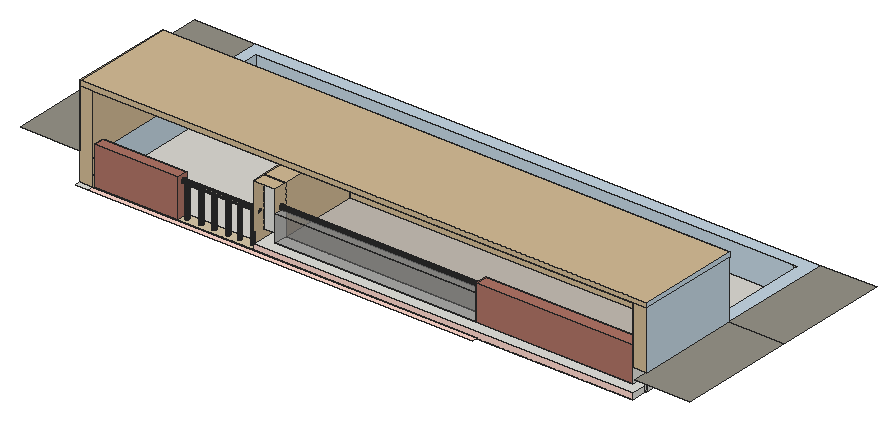
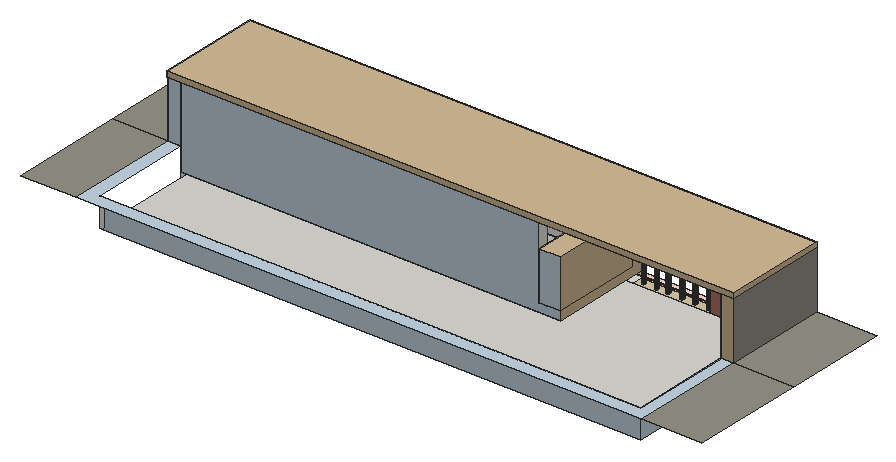
# SketchUp Ruby script. Lengths in inches.
U = 1.inch
M = Sketchup.active_model
def pt(a) = Geom::Point3d.new(a.map { |v| v * U })
def face(e, loops, mat)
  f = e.add_face(loops[0].map { |a| pt(a) })
  loops[1..].each { |l| e.add_face(l.map { |a| pt(a) }).erase! }
  f.material = f.back_material = mat if mat
  f
end
# faces: each face lists its corners as indices into pts; further lists are holes
def faces(e, pts, list, mat = nil) = list.each { |f| face(e, (f[0].is_a?(Array) ? f : [f]).map { |l| l.map { |i| pts[i] } }, mat) }
# xy, xz, yz: faces in a plane at the given z, y or x. An outline is a flat list of corners, or four numbers for a rectangle; further outlines are holes
def ring(l) = l.size == 4 ? [[l[0], l[1]], [l[2], l[1]], [l[2], l[3]], [l[0], l[3]]] : l.each_slice(2).to_a
def flat(e, list, mat, &to3) = list.each { |f| face(e, (f[0].is_a?(Array) ? f : [f]).map { |l| ring(l).map { |u, v| to3.(u, v) } }, mat) }
def xy(e, z, list, mat = nil) = flat(e, list, mat) { |x, y| [x, y, z] }
def xz(e, y, list, mat = nil) = flat(e, list, mat) { |x, z| [x, y, z] }
def yz(e, x, list, mat = nil) = flat(e, list, mat) { |y, z| [x, y, z] }
def lines(e, pts, list) = list.each { |a, b| e.add_line(pt(pts[a]), pt(pts[b])) }
# prism: a flat outline (further loops are holes) pulled along v
def prism(e, loops, v, mat = nil)
  f = face(e, loops, mat); d = Geom::Vector3d.new(v.map { |x| x * U })
  f.pushpull(f.normal.samedirection?(d) ? d.length : -d.length)
end
def box(e, o, s, mat = nil) = prism(e, [[o, [o[0] + s[0], o[1], o[2]], [o[0] + s[0], o[1] + s[1], o[2]], [o[0], o[1] + s[1], o[2]]]], [0, 0, s[2]], mat)
def at(x, y, z, deg = 0) = Geom::Transformation.translation(pt([x, y, z])) * Geom::Transformation.rotation(ORIGIN, Z_AXIS, deg.degrees)
def axes(o, x, y, z) = Geom::Transformation.new([*x, 0, *y, 0, *z, 0, *pt(o).to_a, 1])
def part(name) = M.definitions.add(name)
# library, detail: a bought-in or finely detailed component or shape, given as its bounding box
def library(name, o, s) = part(name).tap { |d| box(d.entities, o, s) }
def detail(e, o, s) = box(e.add_group.entities, o, s)
def put(e, d, t, mat = nil) = e.add_instance(d, t).tap { |i| i.material = mat if mat }
def group(e, t, mat = nil) = e.add_group.tap { |g| g.transformation = t; g.material = mat if mat }.entities
root = M.entities
M.materials.add("[Color B01]").color = [255, 216, 204]
M.materials.add("[Field Rectangle Tile]").color = [196, 189, 179]
M.materials.add("[Field Square Tile]").color = [217, 201, 169]
M.materials.add("[Formica Beige]").color = [211, 187, 149]
M.materials.add("[Formica Graystone]").color = [149, 146, 135]
M.materials.add("[Formica Laminate Dark]").color = [50, 53, 60]
M.materials.add("[Stone Flagstone Ashlar]").color = [175, 116, 102]
M.materials.add("[Terrazzo Light Blue]").color = [196, 214, 227]
M.materials.add("[Terrazzo Tile Light]").color = [219, 217, 210]
M.materials.add("[Translucent Glass Gray]").color = [128, 128, 128]
M.materials["[Translucent Glass Gray]"].alpha = 0.5
xy(root,2381.6875,[[686.75,899.87,2463.34,899.87,2463.34,941.93,1214.38,941.93,1214.38,906.16,686.75,906.16],[686.75,906.16,962.28,941.93],[978.67,919.12,977.11,919.32,975.67,919.92,974.42,920.875,973.47,922.12,972.87,923.57,972.67,925.12,972.87,926.67,973.47,928.12,974.42,929.36,975.67,930.31,977.11,930.91,978.67,931.12,980.22,930.91,981.67,930.31,982.91,929.36,983.86,928.12,984.46,926.67,984.67,925.12,984.46,923.57,983.86,922.12,982.91,920.875,981.67,919.92,980.22,919.32],[1023.73,919.12,1022.18,919.32,1020.73,919.92,1019.49,920.875,1018.53,922.12,1017.93,923.57,1017.73,925.12,1017.93,926.67,1018.53,928.12,1019.49,929.36,1020.73,930.31,1022.18,930.91,1023.73,931.12,1025.28,930.91,1026.73,930.31,1027.97,929.36,1028.92,928.12,1029.52,926.67,1029.73,925.12,1029.52,923.57,1028.92,922.12,1027.97,920.875,1026.73,919.92,1025.28,919.32],[1066.6,919.12,1065.05,919.32,1063.6,919.92,1062.36,920.875,1061.41,922.12,1060.81,923.57,1060.6,925.12,1060.81,926.67,1061.41,928.12,1062.36,929.36,1063.6,930.31,1065.05,930.91,1066.6,931.12,1068.16,930.91,1069.6,930.31,1070.85,929.36,1071.8,928.12,1072.4,926.67,1072.6,925.12,1072.4,923.57,1071.8,922.12,1070.85,920.875,1069.6,919.92,1068.16,919.32],
  [1112.23,919.12,1110.68,919.32,1109.23,919.92,1107.99,920.875,1107.03,922.12,1106.43,923.57,1106.23,925.12,1106.43,926.67,1107.03,928.12,1107.99,929.36,1109.23,930.31,1110.68,930.91,1112.23,931.12,1113.78,930.91,1115.23,930.31,1116.47,929.36,1117.42,928.12,1118.02,926.67,1118.23,925.12,1118.02,923.57,1117.42,922.12,1116.47,920.875,1115.23,919.92,1113.78,919.32],[1149.98,919.12,1148.43,919.32,1146.98,919.92,1145.74,920.875,1144.78,922.12,1144.18,923.57,1143.98,925.12,1144.18,926.67,1144.78,928.12,1145.74,929.36,1146.98,930.31,1148.43,930.91,1149.98,931.12,1151.53,930.91,1152.98,930.31,1154.22,929.36,1155.17,928.12,1155.77,926.67,1155.98,925.12,1155.77,923.57,1155.17,922.12,1154.22,920.875,1152.98,919.92,1151.53,919.32],[1192.73,919.12,1191.18,919.32,1189.73,919.92,1188.49,920.875,1187.53,922.12,1186.93,923.57,1186.73,925.12,1186.93,926.67,1187.53,928.12,1188.49,929.36,1189.73,930.31,1191.18,930.91,1192.73,931.12,1194.28,930.91,1195.73,930.31,1196.97,929.36,1197.92,928.12,1198.52,926.67,1198.73,925.12,1198.52,923.57,1197.92,922.12,1196.97,920.875,1195.73,919.92,1194.28,919.32]])
xy(root,2381.6875,[[[962.28,906.16,1214.38,941.93],[978.67,919.12,977.11,919.32,975.67,919.92,974.42,920.875,973.47,922.12,972.87,923.57,972.67,925.12,972.87,926.67,973.47,928.12,974.42,929.36,975.67,930.31,977.11,930.91,978.67,931.12,980.22,930.91,981.67,930.31,982.91,929.36,983.86,928.12,984.46,926.67,984.67,925.12,984.46,923.57,983.86,922.12,982.91,920.875,981.67,919.92,980.22,919.32],[1192.73,919.12,1191.18,919.32,1189.73,919.92,1188.49,920.875,1187.53,922.12,1186.93,923.57,1186.73,925.12,1186.93,926.67,1187.53,928.12,1188.49,929.36,1189.73,930.31,1191.18,930.91,1192.73,931.12,1194.28,930.91,1195.73,930.31,1196.97,929.36,1197.92,928.12,1198.52,926.67,1198.73,925.12,1198.52,923.57,1197.92,922.12,1196.97,920.875,1195.73,919.92,1194.28,919.32],[1023.73,919.12,1022.18,919.32,1020.73,919.92,1019.49,920.875,1018.53,922.12,1017.93,923.57,1017.73,925.12,1017.93,926.67,1018.53,928.12,1019.49,929.36,1020.73,930.31,1022.18,930.91,1023.73,931.12,1025.28,930.91,1026.73,930.31,1027.97,929.36,1028.92,928.12,1029.52,926.67,1029.73,925.12,1029.52,923.57,1028.92,922.12,1027.97,920.875,1026.73,919.92,1025.28,919.32],[1149.98,919.12,1148.43,919.32,1146.98,919.92,1145.74,920.875,1144.78,922.12,1144.18,923.57,1143.98,925.12,1144.18,926.67,1144.78,928.12,1145.74,929.36,1146.98,930.31,1148.43,930.91,1149.98,931.12,1151.53,930.91,1152.98,930.31,1154.22,929.36,1155.17,928.12,1155.77,926.67,1155.98,925.12,1155.77,923.57,1155.17,922.12,1154.22,920.875,1152.98,919.92,1151.53,919.32],[1066.6,919.12,1065.05,919.32,1063.6,919.92,1062.36,920.875,1061.41,922.12,1060.81,923.57,1060.6,925.12,1060.81,926.67,1061.41,928.12,1062.36,929.36,1063.6,930.31,1065.05,930.91,1066.6,931.12,1068.16,930.91,1069.6,930.31,1070.85,929.36,1071.8,928.12,1072.4,926.67,1072.6,925.12,1072.4,923.57,1071.8,922.12,1070.85,920.875,1069.6,919.92,1068.16,919.32],[1112.23,919.12,1110.68,919.32,1109.23,919.92,1107.99,920.875,1107.03,922.12,1106.43,923.57,1106.23,925.12,1106.43,926.67,1107.03,928.12,1107.99,929.36,1109.23,930.31,1110.68,930.91,1112.23,931.12,1113.78,930.91,1115.23,930.31,1116.47,929.36,1117.42,928.12,1118.02,926.67,1118.23,925.12,1118.02,923.57,1117.42,922.12,1116.47,920.875,1115.23,919.92,1113.78,919.32]]],"[Field Square Tile]")
xy(root,2381.6875,[[686.75,941.93,2463.34,1571.68]],"[Terrazzo Tile Light]")
xy(root,2383.06,[[646.49,880.68,686.75,899.87]])
xy(root,2383.06,[[686.75,880.68,1950.59,899.87]],"[Color B01]")
xy(root,2400.95,[[1215.84,899.87,2463.34,1237.41]])
xy(root,2428.82,[[1286.83,899.87,1946.32,941.93],[1946.32,899.87,2463.34,941.93],[1215.84,941.93,1286.83,1237.41]])
xy(root,2428.82,[[1286.83,941.93,2463.34,1205.85]],"[Field Rectangle Tile]")
xy(root,2476.875,[[2463.34,899.87,2463.34,954.56,2463.77,1237.41,2507.95,1237.41,2507.95,899.87]])
xy(root,2476.875,[[2507.95,849.3125,2688.89,1237.41],[449.56,899.87,646.49,1240.37],[2507.95,1237.41,2688.89,1616.29],[449.56,1240.37,646.49,1616.29]],"[Formica Graystone]")
xy(root,2476.875,[[2463.77,1237.41,2507.95,1237.41,2507.95,1616.29,646.49,1616.29,646.49,1240.37,686.75,1240.37,686.75,1571.68,2464.28,1571.68,2464.28,1257.37,2463.8,1257.37]],"[Terrazzo Light Blue]")
xy(root,2485.1875,[[1023.73,919.12,1025.28,919.32,1026.73,919.92,1027.97,920.875,1028.92,922.12,1029.52,923.57,1029.73,925.12,1029.52,926.67,1028.92,928.12,1027.97,929.36,1026.73,930.31,1025.28,930.91,1023.73,931.12,1022.18,930.91,1020.73,930.31,1019.49,929.36,1018.53,928.12,1017.93,926.67,1017.73,925.12,1017.93,923.57,1018.53,922.12,1019.49,920.875,1020.73,919.92,1022.18,919.32]])
xy(root,2489.1875,[[1149.98,919.12,1151.53,919.32,1152.98,919.92,1154.22,920.875,1155.17,922.12,1155.77,923.57,1155.98,925.12,1155.77,926.67,1155.17,928.12,1154.22,929.36,1152.98,930.31,1151.53,930.91,1149.98,931.12,1148.43,930.91,1146.98,930.31,1145.74,929.36,1144.78,928.12,1144.18,926.67,1143.98,925.12,1144.18,923.57,1144.78,922.12,1145.74,920.875,1146.98,919.92,1148.43,919.32]])
xy(root,2490.375,[[978.67,919.12,980.22,919.32,981.67,919.92,982.91,920.875,983.86,922.12,984.46,923.57,984.67,925.12,984.46,926.67,983.86,928.12,982.91,929.36,981.67,930.31,980.22,930.91,978.67,931.12,977.11,930.91,975.67,930.31,974.42,929.36,973.47,928.12,972.87,926.67,972.67,925.12,972.87,923.57,973.47,922.12,974.42,920.875,975.67,919.92,977.11,919.32]])
xy(root,2492.0625,[[1066.6,919.12,1068.16,919.32,1069.6,919.92,1070.85,920.875,1071.8,922.12,1072.4,923.57,1072.6,925.12,1072.4,926.67,1071.8,928.12,1070.85,929.36,1069.6,930.31,1068.16,930.91,1066.6,931.12,1065.05,930.91,1063.6,930.31,1062.36,929.36,1061.41,928.12,1060.81,926.67,1060.6,925.12,1060.81,923.57,1061.41,922.12,1062.36,920.875,1063.6,919.92,1065.05,919.32]])
xy(root,2492.39,[[1112.23,919.12,1113.78,919.32,1114.35,919.56,1110.1,919.56,1110.68,919.32],[1110.1,919.56,1114.35,919.56,1115.23,919.92,1116.47,920.875,1117.42,922.12,1118.02,923.57,1118.23,925.12,1118.02,926.67,1117.42,928.12,1116.47,929.36,1115.23,930.31,1113.78,930.91,1112.23,931.12,1110.68,930.91,1109.23,930.31,1107.99,929.36,1107.03,928.12,1106.43,926.67,1106.23,925.12,1106.43,923.57,1107.03,922.12,1107.99,920.875,1109.23,919.92]])
xy(root,2492.6875,[[1192.73,919.12,1194.28,919.32,1195.73,919.92,1196.97,920.875,1197.92,922.12,1198.52,923.57,1198.73,925.12,1198.52,926.67,1197.92,928.12,1196.97,929.36,1195.73,930.31,1194.28,930.91,1192.73,931.12,1191.18,930.91,1189.73,930.31,1188.49,929.36,1187.53,928.12,1186.93,926.67,1186.73,925.12,1186.93,923.57,1187.53,922.12,1188.49,920.875,1189.73,919.92,1191.18,919.32]])
xy(root,2506.375,[[686.75,906.16,962.28,941.93]],"[Stone Flagstone Ashlar]")
xy(root,2513.57,[[1286.83,899.87,1946.32,941.93]],"[Translucent Glass Gray]")
xy(root,2542.26,[[1946.32,899.87,2463.34,941.93]],"[Stone Flagstone Ashlar]")
xy(root,2588.07,[[1215.84,899.87,1286.83,941.93],[1215.84,941.93,1286.83,1237.41]],"[Formica Beige]")
xy(root,2665.875,[[646.49,899.87,686.75,1240.37],[2463.34,899.87,2463.34,954.56,2463.77,1237.41,2507.95,1237.41,2507.95,899.87]])
xy(root,2665.875,[[[686.75,899.87,686.75,1240.37,2507.95,1240.37,2507.95,1237.41,2463.77,1237.41,2463.34,954.56,2463.34,899.87],[1286.83,1205.85,2463.34,1237.41]]],"[Terrazzo Tile Light]")
xy(root,2683.3125,[[646.49,899.87,2507.95,1240.37]],"[Formica Beige]")
xz(root,899.87,[[686.75,2381.6875,1215.84,2383.06],[1215.84,2381.6875,1950.59,2383.06]])
xz(root,899.87,[[1950.59,2381.6875,2463.34,2381.6875,2463.34,2400.95,1215.84,2400.95,1215.84,2383.06,1950.59,2383.06]],"[Color B01]")
xz(root,899.87,[[646.49,2383.06,686.75,2665.875],[2463.34,2476.875,2507.95,2665.875],[646.49,2665.875,2507.95,2683.3125]],"[Formica Beige]")
xz(root,899.87,[[1946.32,2428.82,2463.34,2542.26]],"[Stone Flagstone Ashlar]")
xz(root,899.87,[[1286.83,2428.82,1946.32,2513.57]],"[Translucent Glass Gray]")
xz(root,906.16,[[686.75,2381.6875,962.28,2506.375]],"[Stone Flagstone Ashlar]")
xz(root,941.93,[[1215.84,2428.82,1286.83,2588.07]])
xz(root,941.93,[[686.75,2381.6875,962.28,2506.375],[1946.32,2428.82,2463.34,2542.26]],"[Stone Flagstone Ashlar]")
xz(root,941.93,[[1286.83,2428.82,1946.32,2513.57]],"[Translucent Glass Gray]")
xz(root,1205.85,[[1286.83,2428.82,2463.34,2665.875]],"[Formica Beige]")
xz(root,1237.41,[[1215.84,2400.95,1215.84,2428.82,1286.83,2428.82,1286.83,2665.875,2463.34,2665.875,2463.34,2400.95],[1215.84,2428.82,1286.83,2588.07],[2463.77,2476.875,2507.95,2665.875]],"[Terrazzo Light Blue]")
xz(root,1240.37,[[646.49,2476.875,686.75,2665.875],[646.49,2665.875,2507.95,2683.3125]],"[Formica Beige]")
xz(root,1571.68,[[2448.8,2381.6875,2463.34,2476.875]])
xz(root,1571.68,[[686.75,2381.6875,2448.8,2476.875]],"[Terrazzo Light Blue]")
yz(root,646.49,[[899.87,2665.875,1240.37,2683.3125]],"[Formica Beige]")
yz(root,646.49,[[899.87,2476.875,1240.37,2665.875]],"[Formica Graystone]")
yz(root,686.75,[[906.16,2381.6875,941.93,2506.375],[941.93,2381.6875,952.49,2476.875]])
yz(root,686.75,[[899.87,2381.6875,906.16,2381.6875,906.16,2506.375,941.93,2506.375,941.93,2476.875,1240.37,2476.875,1240.37,2665.875,899.87,2665.875]],"[Formica Beige]")
yz(root,686.75,[[952.49,2381.6875,1571.68,2476.875]],"[Terrazzo Light Blue]")
yz(root,962.28,[[925.78,2481.61,923.92,2481.85,922.19,2482.57,920.7,2483.71,919.56,2485.2,918.84,2486.9375,918.6,2488.8,918.84,2490.66,919.56,2492.39,920.7,2493.88,922.19,2495.02,923.92,2495.74,925.78,2495.98,927.64,2495.74,929.38,2495.02,930.87,2493.88,932.01,2492.39,932.73,2490.66,932.97,2488.8,932.73,2486.9375,932.01,2485.2,930.87,2483.71,929.38,2482.57,927.64,2481.85]])
yz(root,962.28,[[[906.16,2381.6875,941.93,2506.375],[925.78,2481.61,923.92,2481.85,922.19,2482.57,920.7,2483.71,919.56,2485.2,918.84,2486.9375,918.6,2488.8,918.84,2490.66,919.56,2492.39,920.7,2493.88,922.19,2495.02,923.92,2495.74,925.78,2495.98,927.64,2495.74,929.38,2495.02,930.87,2493.88,932.01,2492.39,932.73,2490.66,932.97,2488.8,932.73,2486.9375,932.01,2485.2,930.87,2483.71,929.38,2482.57,927.64,2481.85]]],"[Stone Flagstone Ashlar]")
yz(root,1215.84,[[[899.87,2400.95,899.87,2588.07,941.93,2588.07,941.93,2428.82,1237.41,2428.82,1237.41,2400.95],[925.78,2481.61,927.64,2481.85,929.38,2482.57,930.87,2483.71,932.01,2485.2,932.73,2486.9375,932.97,2488.8,932.73,2490.66,932.01,2492.39,930.87,2493.88,929.38,2495.02,927.64,2495.74,925.78,2495.98,923.92,2495.74,922.19,2495.02,920.7,2493.88,919.56,2492.39,918.84,2490.66,918.6,2488.8,918.84,2486.9375,919.56,2485.2,920.7,2483.71,922.19,2482.57,923.92,2481.85]],[941.93,2428.82,1237.41,2588.07]],"[Formica Beige]")
yz(root,1286.83,[[899.87,2428.82,941.93,2513.57],[1205.85,2428.82,1237.41,2588.07],[920.9,2521.24,919.33,2521.45,917.87,2522.06,916.61,2523.02,915.65,2524.27,915.05,2525.74,914.84,2527.31,915.05,2528.875,915.65,2530.34,916.61,2531.59,917.87,2532.56,919.33,2533.16,920.9,2533.37,922.47,2533.16,923.93,2532.56,925.1875,2531.59,926.15,2530.34,926.76,2528.875,926.96,2527.31,926.76,2525.74,926.15,2524.27,925.1875,2523.02,923.93,2522.06,922.47,2521.45],[1205.85,2588.07,1237.41,2665.875]])
yz(root,1286.83,[[941.93,2428.82,1205.85,2588.07],[[899.87,2513.57,941.93,2588.07],[920.9,2521.24,919.33,2521.45,917.87,2522.06,916.61,2523.02,915.65,2524.27,915.05,2525.74,914.84,2527.31,915.05,2528.875,915.65,2530.34,916.61,2531.59,917.87,2532.56,919.33,2533.16,920.9,2533.37,922.47,2533.16,923.93,2532.56,925.1875,2531.59,926.15,2530.34,926.76,2528.875,926.96,2527.31,926.76,2525.74,926.15,2524.27,925.1875,2523.02,923.93,2522.06,922.47,2521.45]]],"[Formica Beige]")
yz(root,1946.32,[[899.87,2428.82,941.93,2513.57]])
yz(root,1946.32,[[[899.87,2513.57,941.93,2542.26],[920.9,2521.24,919.33,2521.45,917.87,2522.06,916.61,2523.02,915.65,2524.27,915.05,2525.74,914.84,2527.31,915.05,2528.875,915.65,2530.34,916.61,2531.59,917.87,2532.56,919.33,2533.16,920.9,2533.37,922.47,2533.16,923.93,2532.56,925.1875,2531.59,926.15,2530.34,926.76,2528.875,926.96,2527.31,926.76,2525.74,926.15,2524.27,925.1875,2523.02,923.93,2522.06,922.47,2521.45]]],"[Stone Flagstone Ashlar]")
yz(root,2463.34,[[899.87,2381.6875,941.93,2400.95],[941.93,2381.6875,952.49,2400.95],[952.49,2381.6875,954.56,2400.95],[954.56,2381.6875,1237.41,2400.95],[954.56,2400.95,1237.41,2400.95,1237.41,2665.875,1205.85,2665.875,1205.85,2428.82,954.56,2428.82],
  [899.87,2428.82,941.93,2476.875],[941.93,2428.82,952.49,2476.875],[952.49,2428.82,954.56,2476.875],[899.87,2476.875,941.93,2542.26]])
yz(root,2463.34,[[941.93,2476.875,952.49,2665.875],[952.49,2476.875,954.56,2665.875],[899.87,2542.26,941.93,2665.875]],"[Formica Beige]")
yz(root,2507.95,[[899.87,2476.875,1237.41,2665.875],[899.87,2665.875,1240.37,2683.3125]],"[Terrazzo Light Blue]")
p = [[977.11,919.32,2381.6875],[978.67,919.12,2381.6875],[978.67,919.12,2490.375],[977.11,919.32,2490.375],[980.22,919.32,2381.6875],[980.22,919.32,2490.375],
  [1022.18,919.32,2381.6875],[1023.73,919.12,2381.6875],[1023.73,919.12,2485.1875],[1022.18,919.32,2485.1875],[1025.28,919.32,2381.6875],[1025.28,919.32,2485.1875],
  [1065.05,919.32,2381.6875],[1066.6,919.12,2381.6875],[1066.6,919.12,2492.0625],[1065.05,919.32,2492.0625],[1068.16,919.32,2381.6875],[1068.16,919.32,2492.0625],
  [1110.68,919.32,2381.6875],[1112.23,919.12,2381.6875],[1112.23,919.12,2492.39],[1110.68,919.32,2492.39],[1113.78,919.32,2381.6875],[1113.78,919.32,2492.39],
  [1148.43,919.32,2381.6875],[1149.98,919.12,2381.6875],[1149.98,919.12,2489.1875],[1148.43,919.32,2489.1875],[1151.53,919.32,2381.6875],[1151.53,919.32,2489.1875],
  [1191.18,919.32,2381.6875],[1192.73,919.12,2381.6875],[1192.73,919.12,2492.6875],[1191.18,919.32,2492.6875],[1194.28,919.32,2381.6875],[1194.28,919.32,2492.6875],
  [975.67,919.92,2381.6875],[975.67,919.92,2490.375],[981.67,919.92,2381.6875],[981.67,919.92,2490.375],[1020.73,919.92,2381.6875],[1020.73,919.92,2485.1875],
  [1026.73,919.92,2381.6875],[1026.73,919.92,2485.1875],[1063.6,919.92,2381.6875],[1063.6,919.92,2492.0625],[1069.6,919.92,2381.6875],[1069.6,919.92,2492.0625],
  [1109.23,919.92,2381.6875],[1110.1,919.56,2492.39],[1109.23,919.92,2492.39],[1115.23,919.92,2381.6875],[1115.23,919.92,2492.39],[1114.35,919.56,2492.39],
  [1146.98,919.92,2381.6875],[1146.98,919.92,2489.1875],[1152.98,919.92,2381.6875],[1152.98,919.92,2489.1875],[1189.73,919.92,2381.6875],[1189.73,919.92,2492.6875],
  [1195.73,919.92,2381.6875],[1195.73,919.92,2492.6875],[974.42,920.875,2381.6875],[974.42,920.875,2490.375],[982.91,920.875,2381.6875],[982.91,920.875,2490.375],
  [1019.49,920.875,2381.6875],[1019.49,920.875,2485.1875],[1027.97,920.875,2381.6875],[1027.97,920.875,2485.1875],[1062.36,920.875,2381.6875],[1062.36,920.875,2492.0625],
  [1070.85,920.875,2381.6875],[1070.85,920.875,2492.0625],[1107.99,920.875,2381.6875],[1107.99,920.875,2492.39],[1116.47,920.875,2381.6875],[1116.47,920.875,2492.39],
  [1145.74,920.875,2381.6875],[1145.74,920.875,2489.1875],[1154.22,920.875,2381.6875],[1154.22,920.875,2489.1875],[1188.49,920.875,2381.6875],[1188.49,920.875,2492.6875],
  [1196.97,920.875,2381.6875],[1196.97,920.875,2492.6875],[973.47,922.12,2381.6875],[973.47,922.12,2490.375],[983.86,922.12,2381.6875],[983.86,922.12,2490.375],
  [1018.53,922.12,2381.6875],[1018.53,922.12,2485.1875],[1028.92,922.12,2381.6875],[1028.92,922.12,2485.1875],[1061.41,922.12,2381.6875],[1061.41,922.12,2492.0625],
  [1071.8,922.12,2381.6875],[1071.8,922.12,2492.0625],[1107.03,922.12,2381.6875],[1107.03,922.12,2492.39],[1117.42,922.12,2381.6875],[1117.42,922.12,2492.39],
  [1144.78,922.12,2381.6875],[1144.78,922.12,2489.1875],[1155.17,922.12,2381.6875],[1155.17,922.12,2489.1875],[1187.53,922.12,2381.6875],[1187.53,922.12,2492.6875],
  [1197.92,922.12,2381.6875],[1197.92,922.12,2492.6875],[972.87,923.57,2381.6875],[972.87,923.57,2490.375],[984.46,923.57,2381.6875],[984.46,923.57,2490.375],
  [1017.93,923.57,2381.6875],[1017.93,923.57,2485.1875],[1029.52,923.57,2381.6875],[1029.52,923.57,2485.1875],[1060.81,923.57,2381.6875],[1060.81,923.57,2492.0625],
  [1072.4,923.57,2381.6875],[1072.4,923.57,2492.0625],[1106.43,923.57,2381.6875],[1106.43,923.57,2492.39],[1118.02,923.57,2381.6875],[1118.02,923.57,2492.39],
  [1144.18,923.57,2381.6875],[1144.18,923.57,2489.1875],[1155.77,923.57,2381.6875],[1155.77,923.57,2489.1875],[1186.93,923.57,2381.6875],[1186.93,923.57,2492.6875],
  [1198.52,923.57,2381.6875],[1198.52,923.57,2492.6875],[972.67,925.12,2381.6875],[972.67,925.12,2490.375],[984.67,925.12,2381.6875],[984.67,925.12,2490.375],
  [1017.73,925.12,2381.6875],[1017.73,925.12,2485.1875],[1029.73,925.12,2381.6875],[1029.73,925.12,2485.1875],[1060.6,925.12,2381.6875],[1060.6,925.12,2492.0625],
  [1072.6,925.12,2381.6875],[1072.6,925.12,2492.0625],[1106.23,925.12,2381.6875],[1106.23,925.12,2492.39],[1118.23,925.12,2381.6875],[1118.23,925.12,2492.39],
  [1143.98,925.12,2381.6875],[1143.98,925.12,2489.1875],[1155.98,925.12,2381.6875],[1155.98,925.12,2489.1875],[1186.73,925.12,2381.6875],[1186.73,925.12,2492.6875],
  [1198.73,925.12,2381.6875],[1198.73,925.12,2492.6875],[972.87,926.67,2381.6875],[972.87,926.67,2490.375],[984.46,926.67,2381.6875],[984.46,926.67,2490.375],
  [1017.93,926.67,2381.6875],[1017.93,926.67,2485.1875],[1029.52,926.67,2381.6875],[1029.52,926.67,2485.1875],[1060.81,926.67,2381.6875],[1060.81,926.67,2492.0625],
  [1072.4,926.67,2381.6875],[1072.4,926.67,2492.0625],[1106.43,926.67,2381.6875],[1106.43,926.67,2492.39],[1118.02,926.67,2381.6875],[1118.02,926.67,2492.39],
  [1144.18,926.67,2381.6875],[1144.18,926.67,2489.1875],[1155.77,926.67,2381.6875],[1155.77,926.67,2489.1875],[1186.93,926.67,2381.6875],[1186.93,926.67,2492.6875],
  [1198.52,926.67,2381.6875],[1198.52,926.67,2492.6875],[973.47,928.12,2381.6875],[973.47,928.12,2490.375],[983.86,928.12,2381.6875],[983.86,928.12,2490.375],
  [1018.53,928.12,2381.6875],[1018.53,928.12,2485.1875],[1028.92,928.12,2381.6875],[1028.92,928.12,2485.1875],[1061.41,928.12,2381.6875],[1061.41,928.12,2492.0625],
  [1071.8,928.12,2381.6875],[1071.8,928.12,2492.0625],[1107.03,928.12,2381.6875],[1107.03,928.12,2492.39],[1117.42,928.12,2381.6875],[1117.42,928.12,2492.39],
  [1144.78,928.12,2381.6875],[1144.78,928.12,2489.1875],[1155.17,928.12,2381.6875],[1155.17,928.12,2489.1875],[1187.53,928.12,2381.6875],[1187.53,928.12,2492.6875],
  [1197.92,928.12,2381.6875],[1197.92,928.12,2492.6875],[974.42,929.36,2381.6875],[974.42,929.36,2490.375],[982.91,929.36,2381.6875],[982.91,929.36,2490.375],
  [1019.49,929.36,2381.6875],[1019.49,929.36,2485.1875],[1027.97,929.36,2381.6875],[1027.97,929.36,2485.1875],[1062.36,929.36,2381.6875],[1062.36,929.36,2492.0625],
  [1070.85,929.36,2381.6875],[1070.85,929.36,2492.0625],[1107.99,929.36,2381.6875],[1107.99,929.36,2492.39],[1116.47,929.36,2381.6875],[1116.47,929.36,2492.39],
  [1145.74,929.36,2381.6875],[1145.74,929.36,2489.1875],[1154.22,929.36,2381.6875],[1154.22,929.36,2489.1875],[1188.49,929.36,2381.6875],[1188.49,929.36,2492.6875],
  [1196.97,929.36,2381.6875],[1196.97,929.36,2492.6875],[975.67,930.31,2381.6875],[975.67,930.31,2490.375],[981.67,930.31,2381.6875],[981.67,930.31,2490.375],
  [1020.73,930.31,2381.6875],[1020.73,930.31,2485.1875],[1026.73,930.31,2381.6875],[1026.73,930.31,2485.1875],[1063.6,930.31,2381.6875],[1063.6,930.31,2492.0625],
  [1069.6,930.31,2381.6875],[1069.6,930.31,2492.0625],[1109.23,930.31,2381.6875],[1109.23,930.31,2492.39],[1115.23,930.31,2381.6875],[1115.23,930.31,2492.39],
  [1146.98,930.31,2381.6875],[1146.98,930.31,2489.1875],[1152.98,930.31,2381.6875],[1152.98,930.31,2489.1875],[1189.73,930.31,2381.6875],[1189.73,930.31,2492.6875],
  [1195.73,930.31,2381.6875],[1195.73,930.31,2492.6875],[977.11,930.91,2381.6875],[977.11,930.91,2490.375],[980.22,930.91,2381.6875],[980.22,930.91,2490.375],
  [1022.18,930.91,2381.6875],[1022.18,930.91,2485.1875],[1025.28,930.91,2381.6875],[1025.28,930.91,2485.1875],[1065.05,930.91,2381.6875],[1065.05,930.91,2492.0625],
  [1068.16,930.91,2381.6875],[1068.16,930.91,2492.0625],[1110.68,930.91,2381.6875],[1110.68,930.91,2492.39],[1113.78,930.91,2381.6875],[1113.78,930.91,2492.39],
  [1148.43,930.91,2381.6875],[1148.43,930.91,2489.1875],[1151.53,930.91,2381.6875],[1151.53,930.91,2489.1875],[1191.18,930.91,2381.6875],[1191.18,930.91,2492.6875],
  [1194.28,930.91,2381.6875],[1194.28,930.91,2492.6875],[978.67,931.12,2381.6875],[978.67,931.12,2490.375],[1023.73,931.12,2381.6875],[1023.73,931.12,2485.1875],
  [1066.6,931.12,2381.6875],[1066.6,931.12,2492.0625],[1112.23,931.12,2381.6875],[1112.23,931.12,2492.39],[1149.98,931.12,2381.6875],[1149.98,931.12,2489.1875],
  [1192.73,931.12,2381.6875],[1192.73,931.12,2492.6875],[2463.77,1237.41,2476.875],[2463.34,954.56,2476.875],[2463.34,954.56,2665.875],[2463.77,1237.41,2665.875],
  [962.28,923.92,2481.85],[962.28,925.78,2481.61],[1215.84,925.78,2481.61],[1215.84,923.92,2481.85],[962.28,927.64,2481.85],[1215.84,927.64,2481.85],
  [962.28,922.19,2482.57],[1215.84,922.19,2482.57],[962.28,929.38,2482.57],[1215.84,929.38,2482.57],[962.28,920.7,2483.71],[1215.84,920.7,2483.71],
  [962.28,930.87,2483.71],[1215.84,930.87,2483.71],[962.28,919.56,2485.2],[1215.84,919.56,2485.2],[962.28,932.01,2485.2],[1215.84,932.01,2485.2],
  [962.28,918.84,2486.9375],[1215.84,918.84,2486.9375],[962.28,932.73,2486.9375],[1215.84,932.73,2486.9375],[962.28,918.6,2488.8],[1215.84,918.6,2488.8],
  [962.28,932.97,2488.8],[1215.84,932.97,2488.8],[962.28,918.84,2490.66],[1215.84,918.84,2490.66],[962.28,932.73,2490.66],[1215.84,932.73,2490.66],
  [962.28,919.56,2492.39],[1215.84,919.56,2492.39],[962.28,932.01,2492.39],[1215.84,932.01,2492.39],[962.28,920.7,2493.88],[1215.84,920.7,2493.88],
  [962.28,930.87,2493.88],[1215.84,930.87,2493.88],[962.28,922.19,2495.02],[1215.84,922.19,2495.02],[962.28,929.38,2495.02],[1215.84,929.38,2495.02],
  [962.28,923.92,2495.74],[1215.84,923.92,2495.74],[962.28,927.64,2495.74],[1215.84,927.64,2495.74],[962.28,925.78,2495.98],[1215.84,925.78,2495.98],
  [1286.83,919.33,2521.45],[1286.83,920.9,2521.24],[1946.32,920.9,2521.24],[1946.32,919.33,2521.45],[1286.83,922.47,2521.45],[1946.32,922.47,2521.45],
  [1286.83,917.87,2522.06],[1946.32,917.87,2522.06],[1286.83,923.93,2522.06],[1946.32,923.93,2522.06],[1286.83,916.61,2523.02],[1946.32,916.61,2523.02],
  [1286.83,925.1875,2523.02],[1946.32,925.1875,2523.02],[1286.83,915.65,2524.27],[1946.32,915.65,2524.27],[1286.83,926.15,2524.27],[1946.32,926.15,2524.27],
  [1286.83,915.05,2525.74],[1946.32,915.05,2525.74],[1286.83,926.76,2525.74],[1946.32,926.76,2525.74],[1286.83,914.84,2527.31],[1946.32,914.84,2527.31],
  [1286.83,926.96,2527.31],[1946.32,926.96,2527.31],[1286.83,915.05,2528.875],[1946.32,915.05,2528.875],[1286.83,926.76,2528.875],[1946.32,926.76,2528.875],
  [1286.83,915.65,2530.34],[1946.32,915.65,2530.34],[1286.83,926.15,2530.34],[1946.32,926.15,2530.34],[1286.83,916.61,2531.59],[1946.32,916.61,2531.59],
  [1286.83,925.1875,2531.59],[1946.32,925.1875,2531.59],[1286.83,917.87,2532.56],[1946.32,917.87,2532.56],[1286.83,923.93,2532.56],[1946.32,923.93,2532.56],
  [1286.83,919.33,2533.16],[1946.32,919.33,2533.16],[1286.83,922.47,2533.16],[1946.32,922.47,2533.16],[1286.83,920.9,2533.37],[1946.32,920.9,2533.37]]
faces(root,p,[[0,1,2,3],[1,4,5,2],[6,7,8,9],[7,10,11,8],[12,13,14,15],[13,16,17,14],[18,19,20,21],[19,22,23,20],
  [24,25,26,27],[25,28,29,26],[30,31,32,33],[31,34,35,32],[36,0,3,37],[4,38,39,5],[40,6,9,41],[10,42,43,11],
  [44,12,15,45],[16,46,47,17],[48,18,21,49,50],[22,51,52,53,23],[54,24,27,55],[28,56,57,29],[58,30,33,59],[34,60,61,35],
  [62,36,37,63],[38,64,65,39],[66,40,41,67],[42,68,69,43],[70,44,45,71],[46,72,73,47],[74,48,50,75],[51,76,77,52],
  [78,54,55,79],[56,80,81,57],[82,58,59,83],[60,84,85,61],[86,62,63,87],[64,88,89,65],[90,66,67,91],[68,92,93,69],
  [94,70,71,95],[72,96,97,73],[98,74,75,99],[76,100,101,77],[102,78,79,103],[80,104,105,81],[106,82,83,107],[84,108,109,85],
  [110,86,87,111],[88,112,113,89],[114,90,91,115],[92,116,117,93],[118,94,95,119],[96,120,121,97],[122,98,99,123],[100,124,125,101],
  [126,102,103,127],[104,128,129,105],[130,106,107,131],[108,132,133,109],[134,110,111,135],[112,136,137,113],[138,114,115,139],[116,140,141,117],
  [142,118,119,143],[120,144,145,121],[146,122,123,147],[124,148,149,125],[150,126,127,151],[128,152,153,129],[154,130,131,155],[132,156,157,133],
  [158,134,135,159],[136,160,161,137],[162,138,139,163],[140,164,165,141],[166,142,143,167],[144,168,169,145],[170,146,147,171],[148,172,173,149],
  [174,150,151,175],[152,176,177,153],[178,154,155,179],[156,180,181,157],[182,158,159,183],[160,184,185,161],[186,162,163,187],[164,188,189,165],
  [190,166,167,191],[168,192,193,169],[194,170,171,195],[172,196,197,173],[198,174,175,199],[176,200,201,177],[202,178,179,203],[180,204,205,181],
  [206,182,183,207],[184,208,209,185],[210,186,187,211],[188,212,213,189],[214,190,191,215],[192,216,217,193],[218,194,195,219],[196,220,221,197],
  [222,198,199,223],[200,224,225,201],[226,202,203,227],[204,228,229,205],[230,206,207,231],[208,232,233,209],[234,210,211,235],[212,236,237,213],
  [238,214,215,239],[216,240,241,217],[242,218,219,243],[220,244,245,221],[246,222,223,247],[224,248,249,225],[250,226,227,251],[228,252,253,229],
  [254,230,231,255],[232,256,257,233],[258,234,235,259],[236,260,261,237],[262,238,239,263],[240,264,265,241],[266,242,243,267],[244,268,269,245],
  [270,246,247,271],[248,272,273,249],[274,250,251,275],[252,276,277,253],[278,254,255,279],[256,278,279,257],[280,258,259,281],[260,280,281,261],
  [282,262,263,283],[264,282,283,265],[284,266,267,285],[268,284,285,269],[286,270,271,287],[272,286,287,273],[288,274,275,289],[276,288,289,277],
  [294,295,296,297],[295,298,299,296],[300,294,297,301],[298,302,303,299],[304,300,301,305],[302,306,307,303],[308,304,305,309],[306,310,311,307],
  [312,308,309,313],[310,314,315,311],[316,312,313,317],[314,318,319,315],[320,316,317,321],[318,322,323,319],[324,320,321,325,53,49],[322,326,327,323],
  [328,324,49,53,325,329],[326,330,331,327],[332,328,329,333],[330,334,335,331],[336,332,333,337],[334,338,339,335],[340,336,337,341],[338,340,341,339]],"[Formica Graystone]")
faces(root,p,[[290,291,292,293]],"[Formica Beige]")
faces(root,p,[[342,343,344,345],[343,346,347,344],[348,342,345,349],[346,350,351,347],[352,348,349,353],[350,354,355,351],[356,352,353,357],[354,358,359,355],
  [360,356,357,361],[358,362,363,359],[364,360,361,365],[362,366,367,363],[368,364,365,369],[366,370,371,367],[372,368,369,373],[370,374,375,371],
  [376,372,373,377],[374,378,379,375],[380,376,377,381],[378,382,383,379],[384,380,381,385],[382,386,387,383],[388,384,385,389],[386,388,389,387]],"[Formica Laminate Dark]")
